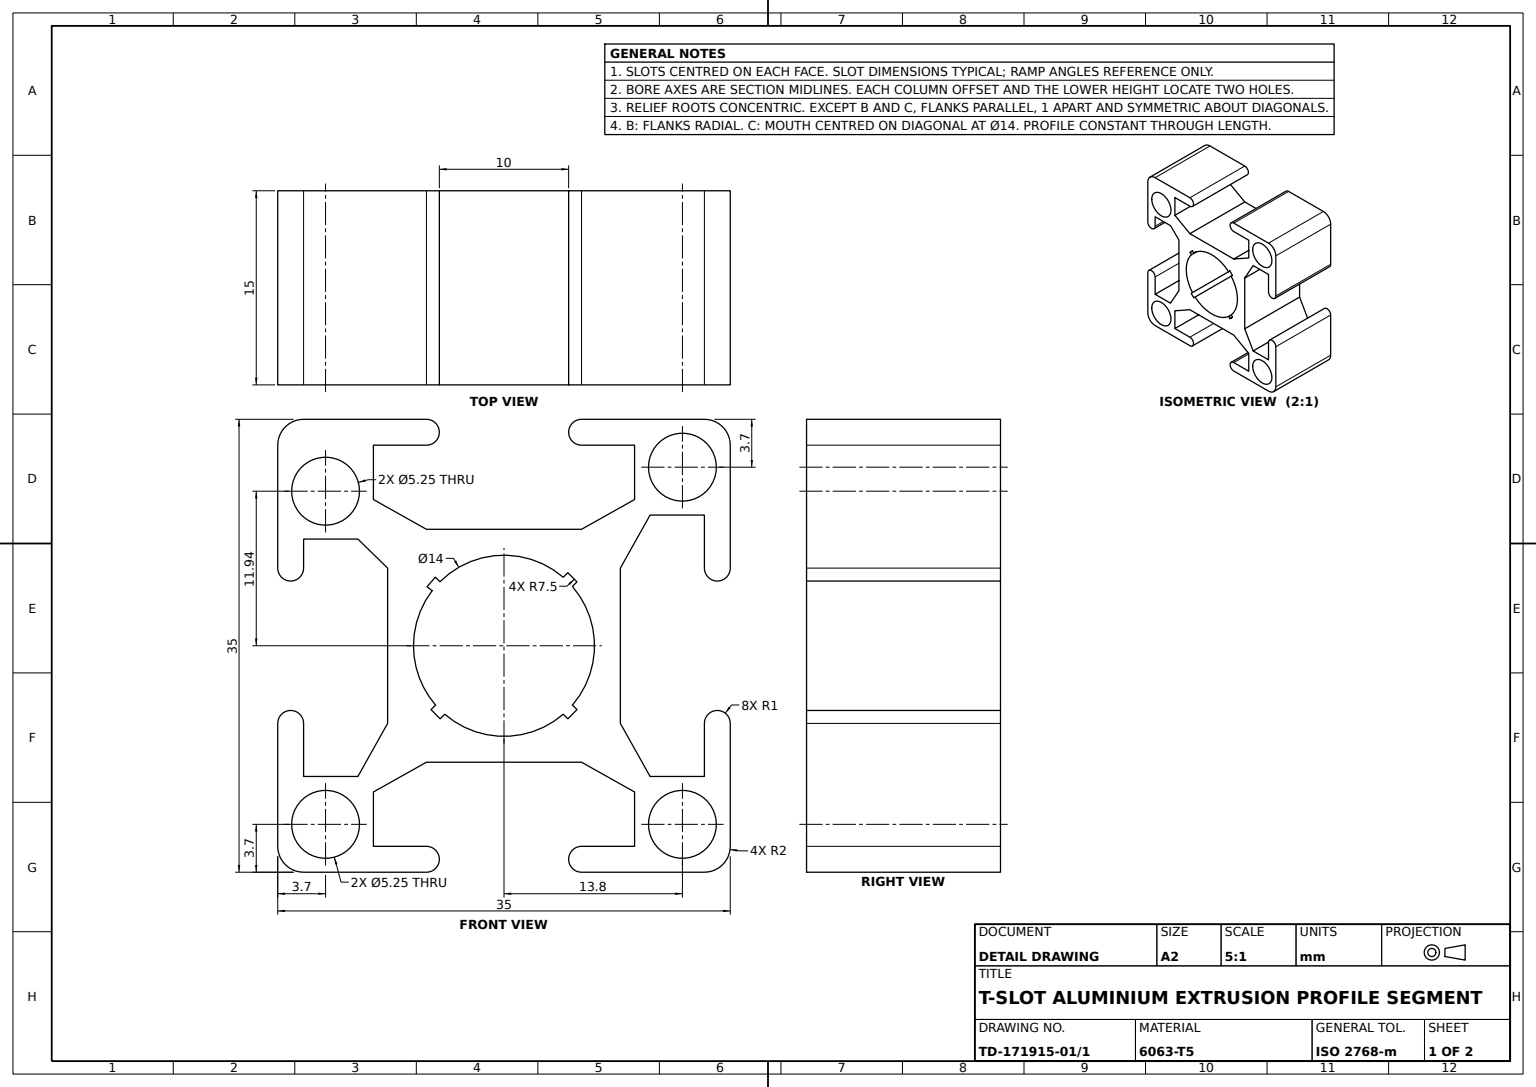
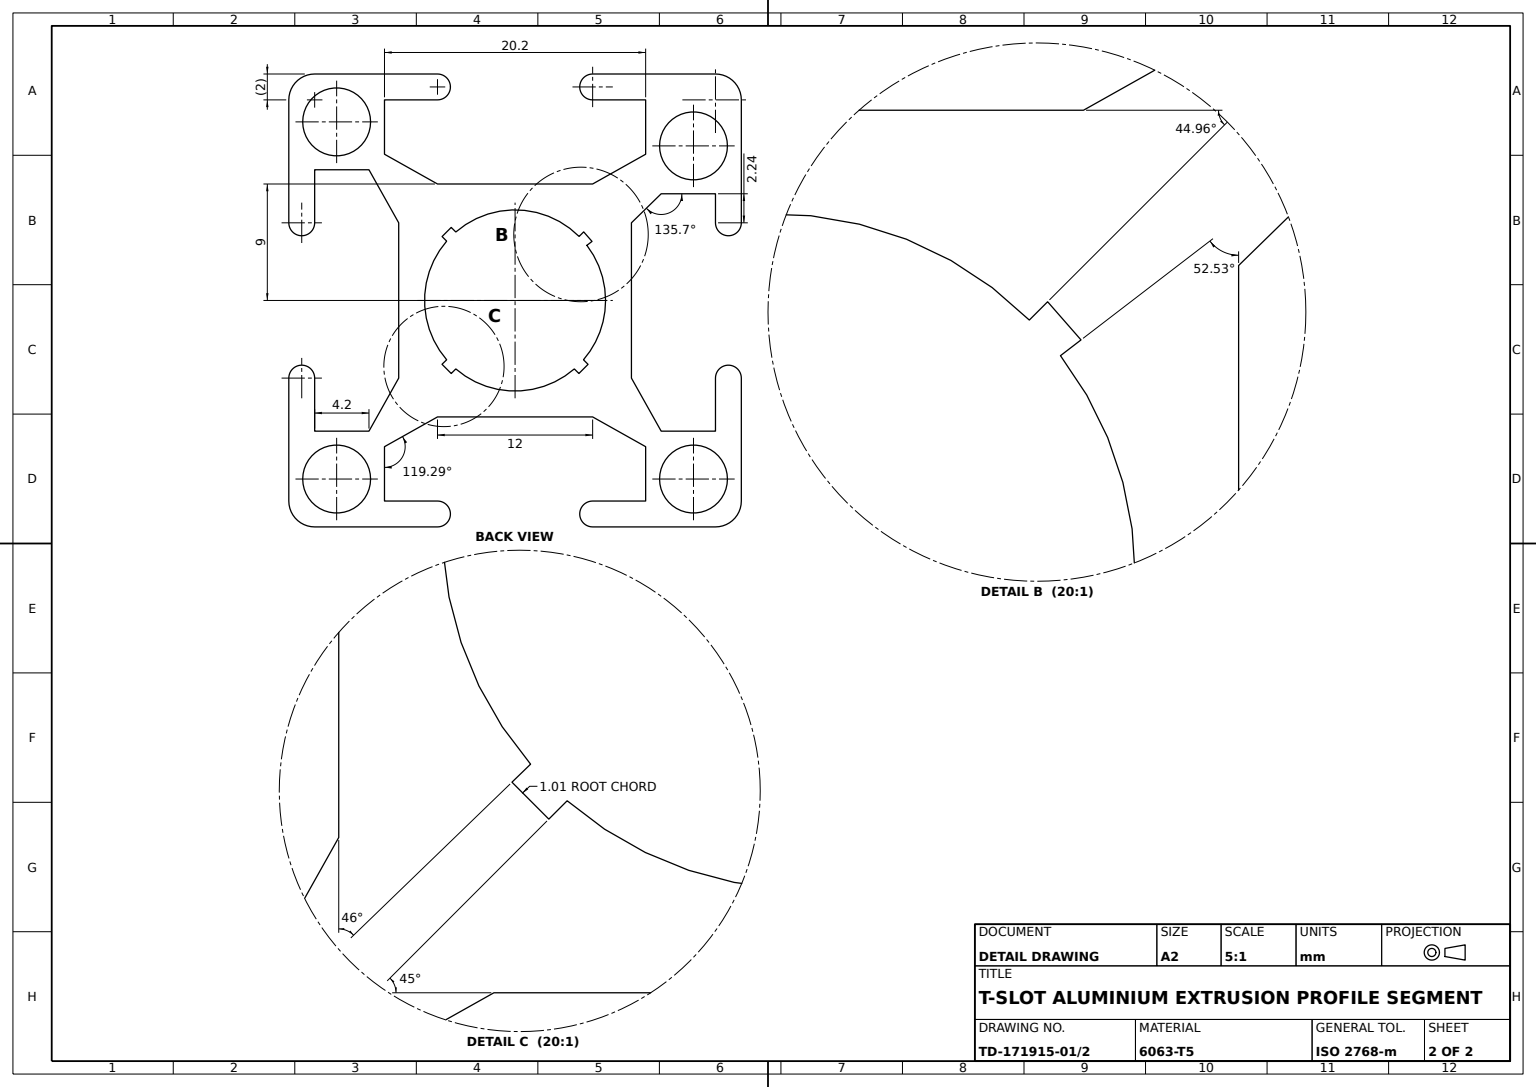
solid
v1 (10.1,-11.3,-7.5)
v2 (10.1,-15.5,-7.5)
e1 v1 v2 LINE
v3 (10.1,-15.5,7.5)
e2 v3 v2 LINE
v4 (10.1,-11.3,7.5)
e3 v4 v3 LINE
e4 v4 v1 LINE
face PLANE(AX(P(10.1,0,7.5),D(1,0,0),D(0,0,-1))) rev [e1 -e2 -e3 e4]
v5 (-4.937949,-5.645056,7.5)
v6 (-4.937949,-5.645056,-7.5)
e5 v5 v6 LINE
v7 (-5.645056,-4.937949,-7.5)
e6 v7 v6 CIRCLE(AX(P(0,0,-7.5),D(0,0,1),D(1,0,0)),7.5)
v8 (-5.645056,-4.937949,7.5)
e7 v8 v7 LINE
e8 v8 v5 CIRCLE(AX(P(0,0,7.5),D(0,0,1),D(1,0,0)),7.5)
face CYL(AX(P(0,0,7.5),D(0,0,-1),D(-1,0,0)),7.5) rev [e5 -e6 -e7 e8]
v9 (4.583551,5.290658,7.5)
v10 (4.937949,5.645056,7.5)
e9 v9 v10 LINE
v11 (4.583551,5.290658,-7.5)
e10 v9 v11 LINE
v12 (4.937949,5.645056,-7.5)
e11 v11 v12 LINE
e12 v10 v12 LINE
face PLANE(AX(P(-0.353553,0.353553,7.5),D(-0.707106781,0.707106781,0),D(-0.707106781,-0.707106781,0))) rev [-e9 e10 e11 -e12]
v13 (-4.952989,4.946504,-7.5)
e13 v11 v13 CIRCLE(AX(P(0,0,-7.5),D(0,0,1),D(1,0,0)),7)
v14 (-4.952989,4.946504,7.5)
e14 v9 v14 CIRCLE(AX(P(0,0,7.5),D(0,0,1),D(1,0,0)),7)
e15 v14 v13 LINE
face CYL(AX(P(0,0,7.5),D(0,0,-1),D(-1,0,0)),7) rev [-e13 -e10 e14 e15]
v15 (5.290453,-4.583787,-7.5)
v16 (5.290658,4.583551,-7.5)
e16 v15 v16 CIRCLE(AX(P(0,0,-7.5),D(0,0,1),D(1,0,0)),7)
v17 (5.290453,-4.583787,7.5)
e17 v17 v15 LINE
v18 (5.290658,4.583551,7.5)
e18 v17 v18 CIRCLE(AX(P(0,0,7.5),D(0,0,1),D(1,0,0)),7)
e19 v18 v16 LINE
face CYL(AX(P(0,0,7.5),D(0,0,-1),D(-1,0,0)),7) rev [-e16 -e17 e18 e19]
v19 (17.5,15.5,7.5)
v20 (17.5,15.5,-7.5)
e20 v19 v20 LINE
v21 (17.5,6,7.5)
e21 v21 v19 LINE
v22 (17.5,6,-7.5)
e22 v21 v22 LINE
e23 v22 v20 LINE
face PLANE(AX(P(17.5,0,7.5),D(-1,0,0),D(0,0,1))) rev [-e20 -e21 e22 e23]
v23 (-6,17.5,7.5)
v24 (-6,17.5,-7.5)
e24 v23 v24 LINE
v25 (-6,15.5,7.5)
e25 v25 v23 CIRCLE(AX(P(-6,16.5,7.5),D(0,0,1),D(1,0,0)),1)
v26 (-6,15.5,-7.5)
e26 v25 v26 LINE
e27 v26 v24 CIRCLE(AX(P(-6,16.5,-7.5),D(0,0,1),D(1,0,0)),1)
face CYL(AX(P(-6,16.5,7.5),D(0,0,-1),D(-1,0,0)),1) [-e24 -e25 e26 e27]
v27 (-10.1,15.5,7.5)
v28 (-10.1,15.5,-7.5)
e28 v27 v28 LINE
e29 v28 v26 LINE
e30 v27 v25 LINE
face PLANE(AX(P(0,15.5,7.5),D(0,1,0),D(0,0,1))) rev [e28 e29 -e26 -e30]
v29 (-11.175,-13.8,7.5)
v30 (-11.175,-13.8,-7.5)
e31 v29 v30 LINE
v31 (-16.425,-13.8,7.5)
e32 v29 v31 CIRCLE(AX(P(-13.8,-13.8,7.5),D(0,0,1),D(1,0,0)),2.625)
v32 (-16.425,-13.8,-7.5)
e33 v31 v32 LINE
e34 v30 v32 CIRCLE(AX(P(-13.8,-13.8,-7.5),D(0,0,1),D(1,0,0)),2.625)
face CYL(AX(P(-13.8,-13.8,7.5),D(0,0,-1),D(-1,0,0)),2.625) rev [-e31 e32 e33 -e34]
v33 (-5.290658,-4.583551,7.5)
v34 (-5.290658,-4.583551,-7.5)
e35 v33 v34 LINE
e36 v33 v8 LINE
e37 v34 v7 LINE
face PLANE(AX(P(-0.353553,0.353553,7.5),D(0.707106781,-0.707106781,0),D(0.707106781,0.707106781,0))) [-e35 e36 e7 -e37]
v35 (-7,0,-7.5)
e38 v35 v34 CIRCLE(AX(P(0,0,-7.5),D(0,0,1),D(1,0,0)),7)
v36 (-7,0,7.5)
e39 v36 v35 LINE
e40 v36 v33 CIRCLE(AX(P(0,0,7.5),D(0,0,1),D(1,0,0)),7)
face CYL(AX(P(0,0,7.5),D(0,0,-1),D(-1,0,0)),7) rev [e35 -e38 -e39 e40]
v37 (-15.5,-6,7.5)
v38 (-15.5,-6,-7.5)
e41 v37 v38 LINE
v39 (-15.5,-10.1,7.5)
e42 v39 v37 LINE
v40 (-15.5,-10.1,-7.5)
e43 v39 v40 LINE
e44 v40 v38 LINE
face PLANE(AX(P(-15.5,0,7.5),D(-1,0,0),D(0,0,1))) rev [-e41 -e42 e43 e44]
v41 (-9,-6,-7.5)
v42 (-11.3,-10.1,-7.5)
e45 v41 v42 LINE
v43 (-11.3,-10.1,7.5)
e46 v43 v42 LINE
v44 (-9,-6,7.5)
e47 v44 v43 LINE
e48 v44 v41 LINE
face PLANE(AX(P(-4.28552,2.404072,7.5),D(0.872143041,-0.489250974,0),D(0.489250974,0.872143041,0))) rev [e45 -e46 -e47 e48]
v45 (-15.5,6,7.5)
v46 (-15.5,6,-7.5)
e49 v45 v46 LINE
v47 (-17.5,6,7.5)
e50 v47 v45 CIRCLE(AX(P(-16.5,6,7.5),D(0,0,1),D(1,0,0)),1)
v48 (-17.5,6,-7.5)
e51 v47 v48 LINE
e52 v48 v46 CIRCLE(AX(P(-16.5,6,-7.5),D(0,0,1),D(1,0,0)),1)
face CYL(AX(P(-16.5,6,7.5),D(0,0,-1),D(-1,0,0)),1) [-e49 -e50 e51 e52]
v49 (-16.425,11.944179,-7.5)
v50 (-11.175,11.944179,-7.5)
e53 v49 v50 CIRCLE(AX(P(-13.8,11.944179,-7.5),D(0,0,1),D(1,0,0)),2.625)
v51 (-16.425,11.944179,7.5)
e54 v51 v49 LINE
v52 (-11.175,11.944179,7.5)
e55 v51 v52 CIRCLE(AX(P(-13.8,11.944179,7.5),D(0,0,1),D(1,0,0)),2.625)
e56 v52 v50 LINE
face CYL(AX(P(-13.8,11.944179,7.5),D(0,0,-1),D(-1,0,0)),2.625) rev [-e53 -e54 e55 e56]
v53 (16.425,13.8,7.5)
v54 (11.175,13.8,7.5)
e57 v53 v54 CIRCLE(AX(P(13.8,13.8,7.5),D(0,0,1),D(1,0,0)),2.625)
v55 (11.175,13.8,-7.5)
e58 v54 v55 LINE
v56 (16.425,13.8,-7.5)
e59 v56 v55 CIRCLE(AX(P(13.8,13.8,-7.5),D(0,0,1),D(1,0,0)),2.625)
e60 v53 v56 LINE
face CYL(AX(P(13.8,13.8,7.5),D(0,0,-1),D(-1,0,0)),2.625) rev [e57 e58 -e59 -e60]
v57 (6,15.5,7.5)
v58 (6,15.5,-7.5)
e61 v57 v58 LINE
v59 (5,16.5,7.5)
e62 v59 v57 CIRCLE(AX(P(6,16.5,7.5),D(0,0,1),D(1,0,0)),1)
v60 (5,16.5,-7.5)
e63 v59 v60 LINE
e64 v60 v58 CIRCLE(AX(P(6,16.5,-7.5),D(0,0,1),D(1,0,0)),1)
face CYL(AX(P(6,16.5,7.5),D(0,0,-1),D(-1,0,0)),1) [-e61 -e62 e63 e64]
v61 (5.650606,-4.931597,7.5)
v62 (5.650606,-4.931597,-7.5)
e65 v61 v62 LINE
v63 (4.937949,-5.645056,-7.5)
e66 v63 v62 CIRCLE(AX(P(0,0,-7.5),D(0,0,1),D(1,0,0)),7.5)
v64 (4.937949,-5.645056,7.5)
e67 v64 v63 LINE
e68 v64 v61 CIRCLE(AX(P(0,0,7.5),D(0,0,1),D(1,0,0)),7.5)
face CYL(AX(P(0,0,7.5),D(0,0,-1),D(-1,0,0)),7.5) rev [e65 -e66 -e67 e68]
v65 (6,-15.5,7.5)
v66 (5,-16.5,7.5)
e69 v65 v66 CIRCLE(AX(P(6,-16.5,7.5),D(0,0,1),D(1,0,0)),1)
v67 (6,-15.5,-7.5)
e70 v65 v67 LINE
v68 (5,-16.5,-7.5)
e71 v67 v68 CIRCLE(AX(P(6,-16.5,-7.5),D(0,0,1),D(1,0,0)),1)
e72 v66 v68 LINE
face CYL(AX(P(6,-16.5,7.5),D(0,0,-1),D(-1,0,0)),1) [-e69 e70 e71 -e72]
v69 (-17.5,-15.5,7.5)
v70 (-17.5,-15.5,-7.5)
e73 v69 v70 LINE
v71 (-15.5,-17.5,-7.5)
e74 v70 v71 CIRCLE(AX(P(-15.5,-15.5,-7.5),D(0,0,1),D(1,0,0)),2)
v72 (-15.5,-17.5,7.5)
e75 v72 v71 LINE
e76 v69 v72 CIRCLE(AX(P(-15.5,-15.5,7.5),D(0,0,1),D(1,0,0)),2)
face CYL(AX(P(-15.5,-15.5,7.5),D(0,0,-1),D(-1,0,0)),2) [e73 e74 -e75 -e76]
e77 v54 v53 CIRCLE(AX(P(13.8,13.8,7.5),D(0,0,1),D(1,0,0)),2.625)
e78 v55 v56 CIRCLE(AX(P(13.8,13.8,-7.5),D(0,0,1),D(1,0,0)),2.625)
face CYL(AX(P(13.8,13.8,7.5),D(0,0,-1),D(-1,0,0)),2.625) rev [-e58 e77 e60 -e78]
v73 (11.175,-13.8,7.5)
v74 (11.175,-13.8,-7.5)
e79 v73 v74 LINE
v75 (16.425,-13.8,-7.5)
e80 v75 v74 CIRCLE(AX(P(13.8,-13.8,-7.5),D(0,0,1),D(1,0,0)),2.625)
v76 (16.425,-13.8,7.5)
e81 v76 v75 LINE
e82 v76 v73 CIRCLE(AX(P(13.8,-13.8,7.5),D(0,0,1),D(1,0,0)),2.625)
face CYL(AX(P(13.8,-13.8,7.5),D(0,0,-1),D(-1,0,0)),2.625) rev [e79 -e80 -e81 e82]
e83 v3 v65 LINE
e84 v2 v67 LINE
face PLANE(AX(P(0,-15.5,7.5),D(0,-1,0),D(0,0,-1))) rev [-e83 e2 e84 -e70]
v77 (5.645056,4.937949,7.5)
e85 v18 v77 LINE
v78 (5.645056,4.937949,-7.5)
e86 v77 v78 LINE
e87 v16 v78 LINE
face PLANE(AX(P(0.353553,-0.353553,7.5),D(-0.707106781,0.707106781,0),D(-0.707106781,-0.707106781,0))) [e85 e86 -e87 -e19]
v79 (10.1,11.3,7.5)
v80 (10.1,11.3,-7.5)
e88 v79 v80 LINE
v81 (6,9,-7.5)
e89 v81 v80 LINE
v82 (6,9,7.5)
e90 v82 v81 LINE
e91 v82 v79 LINE
face PLANE(AX(P(-2.404072,4.28552,7.5),D(-0.489250974,0.872143041,0),D(-0.872143041,-0.489250974,0))) [e88 -e89 -e90 e91]
v83 (-17.5,-6,7.5)
e92 v83 v69 LINE
v84 (-17.5,-6,-7.5)
e93 v83 v84 LINE
e94 v84 v70 LINE
face PLANE(AX(P(-17.5,0,7.5),D(1,0,0),D(0,1,0))) rev [-e73 -e92 e93 e94]
v85 (6,17.5,7.5)
e95 v85 v59 CIRCLE(AX(P(6,16.5,7.5),D(0,0,1),D(1,0,0)),1)
v86 (6,17.5,-7.5)
e96 v85 v86 LINE
e97 v86 v60 CIRCLE(AX(P(6,16.5,-7.5),D(0,0,1),D(1,0,0)),1)
face CYL(AX(P(6,16.5,7.5),D(0,0,-1),D(-1,0,0)),1) [-e63 -e95 e96 e97]
e98 v78 v12 CIRCLE(AX(P(0,0,-7.5),D(0,0,1),D(1,0,0)),7.5)
e99 v77 v10 CIRCLE(AX(P(0,0,7.5),D(0,0,1),D(1,0,0)),7.5)
face CYL(AX(P(0,0,7.5),D(0,0,-1),D(-1,0,0)),7.5) rev [-e98 -e86 e99 e12]
v87 (-10.1,11.3,7.5)
e100 v87 v27 LINE
v88 (-10.1,11.3,-7.5)
e101 v87 v88 LINE
e102 v88 v28 LINE
face PLANE(AX(P(-10.1,0,7.5),D(-1,0,0),D(0,0,1))) rev [-e28 -e100 e101 e102]
v89 (15.5,-6,7.5)
v90 (15.5,-6,-7.5)
e103 v89 v90 LINE
v91 (17.5,-6,7.5)
e104 v91 v89 CIRCLE(AX(P(16.5,-6,7.5),D(0,0,1),D(1,0,0)),1)
v92 (17.5,-6,-7.5)
e105 v91 v92 LINE
e106 v92 v90 CIRCLE(AX(P(16.5,-6,-7.5),D(0,0,1),D(1,0,0)),1)
face CYL(AX(P(16.5,-6,7.5),D(0,0,-1),D(-1,0,0)),1) [-e103 -e104 e105 e106]
v93 (-15.5,17.5,-7.5)
e107 v24 v93 LINE
v94 (-15.5,17.5,7.5)
e108 v94 v93 LINE
e109 v23 v94 LINE
face PLANE(AX(P(0,17.5,7.5),D(0,-1,0),D(1,0,0))) rev [e24 e107 -e108 -e109]
e110 v73 v76 CIRCLE(AX(P(13.8,-13.8,7.5),D(0,0,1),D(1,0,0)),2.625)
e111 v74 v75 CIRCLE(AX(P(13.8,-13.8,-7.5),D(0,0,1),D(1,0,0)),2.625)
face CYL(AX(P(13.8,-13.8,7.5),D(0,0,-1),D(-1,0,0)),2.625) rev [e110 e81 -e111 -e79]
v95 (15.5,6,7.5)
v96 (15.5,6,-7.5)
e112 v95 v96 LINE
v97 (15.5,10.1,7.5)
e113 v95 v97 LINE
v98 (15.5,10.1,-7.5)
e114 v97 v98 LINE
e115 v96 v98 LINE
face PLANE(AX(P(15.5,0,7.5),D(-1,0,0),D(0,-1,0))) [-e112 e113 e114 -e115]
e116 v38 v84 CIRCLE(AX(P(-16.5,-6,-7.5),D(0,0,1),D(1,0,0)),1)
e117 v37 v83 CIRCLE(AX(P(-16.5,-6,7.5),D(0,0,1),D(1,0,0)),1)
face CYL(AX(P(-16.5,-6,7.5),D(0,0,-1),D(-1,0,0)),1) [e41 e116 -e93 -e117]
v99 (-10.1,-15.5,7.5)
v100 (-10.1,-15.5,-7.5)
e118 v99 v100 LINE
v101 (-10.1,-11.3,-7.5)
e119 v100 v101 LINE
v102 (-10.1,-11.3,7.5)
e120 v102 v101 LINE
e121 v99 v102 LINE
face PLANE(AX(P(-10.1,0,7.5),D(-1,0,0),D(0,0,1))) rev [e118 e119 -e120 -e121]
v103 (9,-6,-7.5)
v104 (11.3,-10.1,-7.5)
e122 v103 v104 LINE
v105 (9,-6,7.5)
e123 v105 v103 LINE
v106 (11.3,-10.1,7.5)
e124 v105 v106 LINE
e125 v106 v104 LINE
face PLANE(AX(P(4.28552,2.404072,7.5),D(0.872143041,0.489250974,0),D(-0.489250974,0.872143041,0))) [-e122 -e123 e124 e125]
e126 v52 v51 CIRCLE(AX(P(-13.8,11.944179,7.5),D(0,0,1),D(1,0,0)),2.625)
e127 v50 v49 CIRCLE(AX(P(-13.8,11.944179,-7.5),D(0,0,1),D(1,0,0)),2.625)
face CYL(AX(P(-13.8,11.944179,7.5),D(0,0,-1),D(-1,0,0)),2.625) rev [e126 e54 -e127 -e56]
e128 v42 v40 LINE
e129 v43 v39 LINE
face PLANE(AX(P(0,-10.1,7.5),D(0,-1,0),D(0,0,-1))) rev [e128 -e43 -e129 e46]
v107 (6,-9,7.5)
v108 (6,-9,-7.5)
e130 v107 v108 LINE
v109 (-6,-9,7.5)
e131 v107 v109 LINE
v110 (-6,-9,-7.5)
e132 v109 v110 LINE
e133 v108 v110 LINE
face PLANE(AX(P(0,-9,7.5),D(0,-1,0),D(0,0,-1))) [-e130 e131 e132 -e133]
v111 (9,6,7.5)
v112 (9,6,-7.5)
e134 v111 v112 LINE
e135 v111 v105 LINE
e136 v112 v103 LINE
face PLANE(AX(P(9,0,7.5),D(1,0,0),D(0,1,0))) [-e134 e135 e123 -e136]
v113 (-5.555627,4.258522,7.5)
v114 (-5.952457,4.562703,7.5)
e137 v113 v114 LINE
v115 (-5.555627,4.258522,-7.5)
e138 v113 v115 LINE
v116 (-5.952457,4.562703,-7.5)
e139 v115 v116 LINE
e140 v114 v116 LINE
face PLANE(AX(P(0,0,7.5),D(-0.608360337,-0.793660948,0),D(0.793660948,-0.608360337,0))) rev [-e137 e138 e139 -e140]
v117 (15.5,17.5,-7.5)
e141 v117 v86 LINE
v118 (15.5,17.5,7.5)
e142 v118 v85 LINE
e143 v118 v117 LINE
face PLANE(AX(P(0,17.5,7.5),D(0,-1,0),D(1,0,0))) rev [e141 -e96 -e142 e143]
v119 (-6,9,7.5)
v120 (-6,9,-7.5)
e144 v119 v120 LINE
e145 v119 v82 LINE
e146 v120 v81 LINE
face PLANE(AX(P(0,9,7.5),D(0,1,0),D(0,0,1))) [-e144 e145 e90 -e146]
v121 (10.1,15.5,7.5)
e147 v79 v121 LINE
v122 (10.1,15.5,-7.5)
e148 v121 v122 LINE
e149 v80 v122 LINE
face PLANE(AX(P(10.1,0,7.5),D(-1,0,0),D(0,0,1))) [e147 e148 -e149 -e88]
v123 (11.3,10.1,-7.5)
e150 v112 v123 LINE
v124 (11.3,10.1,7.5)
e151 v124 v123 LINE
e152 v111 v124 LINE
face PLANE(AX(P(4.28552,-2.404072,7.5),D(-0.872143041,0.489250974,0),D(-0.489250974,-0.872143041,0))) rev [e150 -e151 -e152 e134]
v125 (-5.306774,5.299826,7.5)
e153 v125 v114 CIRCLE(AX(P(0,0,7.5),D(0,0,1),D(1,0,0)),7.5)
v126 (-5.306774,5.299826,-7.5)
e154 v126 v116 CIRCLE(AX(P(0,0,-7.5),D(0,0,1),D(1,0,0)),7.5)
e155 v125 v126 LINE
face CYL(AX(P(0,0,7.5),D(0,0,-1),D(-1,0,0)),7.5) rev [e153 e140 -e154 -e155]
e156 v14 v125 LINE
e157 v13 v126 LINE
face PLANE(AX(P(0,0,7.5),D(-0.706643425,-0.707569834,0),D(0.707569834,-0.706643425,0))) [-e15 e156 e155 -e157]
v127 (6,-17.5,7.5)
v128 (6,-17.5,-7.5)
e158 v127 v128 LINE
e159 v66 v127 CIRCLE(AX(P(6,-16.5,7.5),D(0,0,1),D(1,0,0)),1)
e160 v68 v128 CIRCLE(AX(P(6,-16.5,-7.5),D(0,0,1),D(1,0,0)),1)
face CYL(AX(P(6,-16.5,7.5),D(0,0,-1),D(-1,0,0)),1) [-e158 -e159 e72 e160]
v129 (4.583551,-5.290658,7.5)
e161 v129 v64 LINE
v130 (-4.583551,-5.290658,7.5)
e162 v130 v129 CIRCLE(AX(P(0,0,7.5),D(0,0,1),D(1,0,0)),7)
e163 v130 v5 LINE
e164 v113 v36 CIRCLE(AX(P(0,0,7.5),D(0,0,1),D(1,0,0)),7)
e165 v17 v61 LINE
e166 v31 v29 CIRCLE(AX(P(-13.8,-13.8,7.5),D(0,0,1),D(1,0,0)),2.625)
v131 (15.5,-10.1,7.5)
e167 v89 v131 LINE
e168 v131 v106 LINE
e169 v97 v124 LINE
e170 v95 v21 CIRCLE(AX(P(16.5,6,7.5),D(0,0,1),D(1,0,0)),1)
e171 v19 v118 CIRCLE(AX(P(15.5,15.5,7.5),D(0,0,1),D(1,0,0)),2)
e172 v57 v121 LINE
e173 v119 v87 LINE
v132 (-17.5,15.5,7.5)
e174 v94 v132 CIRCLE(AX(P(-15.5,15.5,7.5),D(0,0,1),D(1,0,0)),2)
e175 v132 v47 LINE
v133 (-15.5,8.244179,7.5)
e176 v133 v45 LINE
v134 (-11.3,8.244179,7.5)
e177 v134 v133 LINE
v135 (-9,6,7.5)
e178 v135 v134 LINE
e179 v44 v135 LINE
v136 (-6,-17.5,7.5)
e180 v72 v136 LINE
v137 (-6,-15.5,7.5)
e181 v136 v137 CIRCLE(AX(P(-6,-16.5,7.5),D(0,0,1),D(1,0,0)),1)
e182 v137 v99 LINE
e183 v109 v102 LINE
e184 v107 v4 LINE
v138 (15.5,-17.5,7.5)
e185 v127 v138 LINE
v139 (17.5,-15.5,7.5)
e186 v138 v139 CIRCLE(AX(P(15.5,-15.5,7.5),D(0,0,1),D(1,0,0)),2)
e187 v139 v91 LINE
face PLANE(AX(P(0,0,7.5),D(0,0,1),D(1,0,0))) [-e55 -e126] [-e161 -e162 e163 -e8 -e36 -e40 -e164 e137 -e153 -e156 -e14 e9 -e99 -e85 -e18 e165 -e68] [-e57 -e77] [-e166 -e32] [-e110 -e82] [e167 e168 -e124 -e135 e152 -e169 -e113 e170 e21 e171 e142 e95 e62 e172 -e147 -e91 -e145 e173 e100 e30 e25 e109 e174 e175 e50 -e176 -e177 -e178 -e179 e47 e129 e42 e117 e92 e76 e180 e181 e182 e121 -e183 -e131 e184 e3 e83 e69 e159 e185 e186 e187 e104]
v140 (-11.3,8.244179,-7.5)
v141 (-15.5,8.244179,-7.5)
e188 v140 v141 LINE
e189 v134 v140 LINE
e190 v133 v141 LINE
face PLANE(AX(P(0,8.244179,7.5),D(0,-1,0),D(0,0,-1))) [-e188 -e189 e177 e190]
v142 (-4.583551,-5.290658,-7.5)
e191 v130 v142 LINE
e192 v142 v6 LINE
face PLANE(AX(P(0.353553,-0.353553,7.5),D(0.707106781,-0.707106781,0),D(0.707106781,0.707106781,0))) rev [-e163 e191 e192 -e5]
e193 v115 v35 CIRCLE(AX(P(0,0,-7.5),D(0,0,1),D(1,0,0)),7)
v143 (4.583551,-5.290658,-7.5)
e194 v142 v143 CIRCLE(AX(P(0,0,-7.5),D(0,0,1),D(1,0,0)),7)
e195 v143 v63 LINE
e196 v15 v62 LINE
e197 v108 v1 LINE
e198 v110 v101 LINE
v144 (-6,-15.5,-7.5)
e199 v144 v100 LINE
v145 (-6,-17.5,-7.5)
e200 v145 v144 CIRCLE(AX(P(-6,-16.5,-7.5),D(0,0,1),D(1,0,0)),1)
e201 v71 v145 LINE
v146 (-9,6,-7.5)
e202 v41 v146 LINE
e203 v146 v140 LINE
e204 v141 v46 LINE
v147 (-17.5,15.5,-7.5)
e205 v147 v48 LINE
e206 v93 v147 CIRCLE(AX(P(-15.5,15.5,-7.5),D(0,0,1),D(1,0,0)),2)
e207 v120 v88 LINE
e208 v58 v122 LINE
e209 v20 v117 CIRCLE(AX(P(15.5,15.5,-7.5),D(0,0,1),D(1,0,0)),2)
e210 v96 v22 CIRCLE(AX(P(16.5,6,-7.5),D(0,0,1),D(1,0,0)),1)
e211 v98 v123 LINE
v148 (15.5,-10.1,-7.5)
e212 v148 v104 LINE
e213 v90 v148 LINE
v149 (17.5,-15.5,-7.5)
e214 v149 v92 LINE
v150 (15.5,-17.5,-7.5)
e215 v150 v149 CIRCLE(AX(P(15.5,-15.5,-7.5),D(0,0,1),D(1,0,0)),2)
e216 v128 v150 LINE
e217 v32 v30 CIRCLE(AX(P(-13.8,-13.8,-7.5),D(0,0,1),D(1,0,0)),2.625)
face PLANE(AX(P(0,0,-7.5),D(0,0,1),D(1,0,0))) rev [e154 -e139 e193 e38 e37 e6 -e192 e194 e195 e66 -e196 e16 e87 e98 -e11 e13 e157] [-e84 -e1 -e197 e133 e198 -e119 -e199 -e200 -e201 -e74 -e94 -e116 -e44 -e128 -e45 e202 e203 e188 e204 -e52 -e205 -e206 -e107 -e27 -e29 -e102 -e207 e146 e89 e149 -e208 -e64 -e97 -e141 -e209 -e23 -e210 e115 e211 -e150 e136 e122 -e212 -e213 -e106 -e214 -e215 -e216 -e160 -e71] [e78 e59] [e80 e111] [e34 e217] [e53 e127]
face PLANE(AX(P(0,10.1,7.5),D(0,-1,0),D(0,0,-1))) [e169 e151 -e211 -e114]
e218 v129 v143 LINE
face PLANE(AX(P(-0.353553,-0.353553,7.5),D(0.707106781,0.707106781,0),D(-0.707106781,0.707106781,0))) [-e195 -e218 e161 e67]
face CYL(AX(P(0,0,7.5),D(0,0,-1),D(-1,0,0)),7) rev [-e138 e164 e39 -e193]
face CYL(AX(P(15.5,15.5,7.5),D(0,0,-1),D(-1,0,0)),2) [-e171 e20 e209 -e143]
e219 v131 v148 LINE
face PLANE(AX(P(0,-10.1,7.5),D(0,-1,0),D(0,0,-1))) rev [-e168 e219 e212 -e125]
face CYL(AX(P(0,0,7.5),D(0,0,-1),D(-1,0,0)),7) rev [-e191 e162 e218 -e194]
face CYL(AX(P(16.5,6,7.5),D(0,0,-1),D(-1,0,0)),1) [-e22 -e170 e112 e210]
face PLANE(AX(P(2.404072,4.28552,7.5),D(-0.489250974,-0.872143041,0),D(0.872143041,-0.489250974,0))) rev [-e173 e144 e207 -e101]
e220 v136 v145 LINE
face PLANE(AX(P(0,-17.5,7.5),D(0,1,0),D(0,0,1))) rev [-e180 e75 e201 -e220]
e221 v132 v147 LINE
face PLANE(AX(P(-17.5,0,7.5),D(1,0,0),D(0,1,0))) rev [e205 -e51 -e175 e221]
e222 v137 v144 LINE
face PLANE(AX(P(0,-15.5,7.5),D(0,-1,0),D(1,0,0))) rev [-e182 e222 e199 -e118]
e223 v135 v146 LINE
face PLANE(AX(P(-1.390365,-1.424949,7.5),D(-0.698367945,-0.715738928,0),D(0.715738928,-0.698367945,0))) [-e223 e178 e189 -e203]
face CYL(AX(P(-6,-16.5,7.5),D(0,0,-1),D(-1,0,0)),1) [e220 e200 -e222 -e181]
face PLANE(AX(P(0.262522,0.271837,7.5),D(0.694673695,0.719325001,0),D(-0.719325001,0.694673695,0))) rev [e17 e196 -e65 -e165]
face PLANE(AX(P(-15.5,0,7.5),D(1,0,0),D(0,0,-1))) [-e190 e176 e49 -e204]
face PLANE(AX(P(-2.404072,-4.28552,7.5),D(0.489250974,0.872143041,0),D(-0.872143041,0.489250974,0))) rev [-e184 e130 e197 -e4]
face CYL(AX(P(-13.8,-13.8,7.5),D(0,0,-1),D(-1,0,0)),2.625) rev [e166 e31 -e217 -e33]
face PLANE(AX(P(-9,0,7.5),D(-1,0,0),D(0,0,1))) [e223 -e202 -e48 e179]
e224 v138 v150 LINE
face PLANE(AX(P(0,-17.5,7.5),D(0,1,0),D(0,0,1))) rev [e216 -e224 -e185 e158]
face CYL(AX(P(-15.5,15.5,7.5),D(0,0,-1),D(-1,0,0)),2) [-e221 -e174 e108 e206]
face PLANE(AX(P(15.5,0,7.5),D(1,0,0),D(0,1,0))) rev [e213 -e219 -e167 e103]
face PLANE(AX(P(2.404072,-4.28552,7.5),D(0.489250974,-0.872143041,0),D(0.872143041,0.489250974,0))) [e120 -e198 -e132 e183]
face PLANE(AX(P(0,15.5,7.5),D(0,1,0),D(-1,0,0))) rev [-e172 e61 e208 -e148]
e225 v139 v149 LINE
face CYL(AX(P(15.5,-15.5,7.5),D(0,0,-1),D(-1,0,0)),2) [-e225 -e186 e224 e215]
face PLANE(AX(P(17.5,0,7.5),D(-1,0,0),D(0,0,1))) rev [-e187 e225 e214 -e105]
